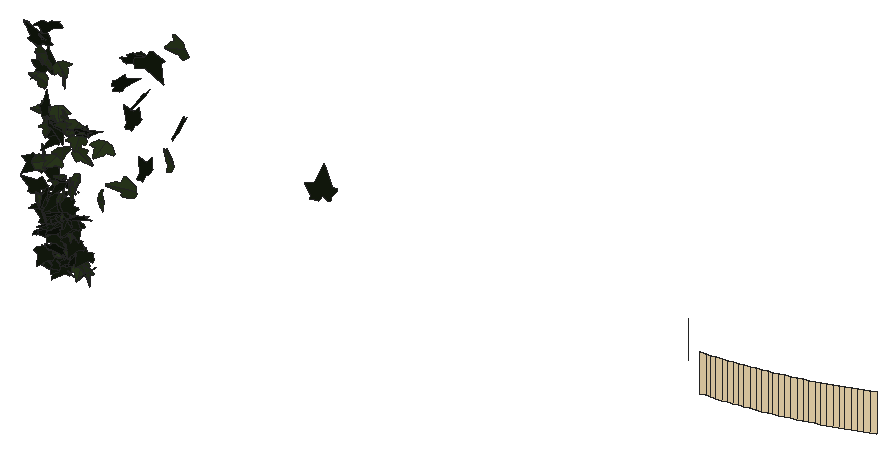
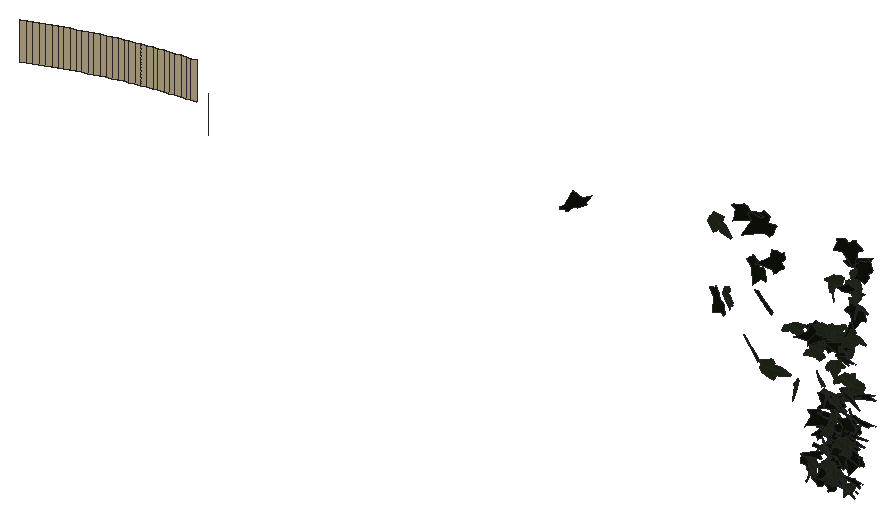
# SketchUp Ruby script. Lengths in inches.
U = 1.inch
M = Sketchup.active_model
def pt(a) = Geom::Point3d.new(a.map { |v| v * U })
def face(e, loops, mat)
  f = e.add_face(loops[0].map { |a| pt(a) })
  loops[1..].each { |l| e.add_face(l.map { |a| pt(a) }).erase! }
  f.material = f.back_material = mat if mat
  f
end
# faces: each face lists its corners as indices into pts; further lists are holes
def faces(e, pts, list, mat = nil) = list.each { |f| face(e, (f[0].is_a?(Array) ? f : [f]).map { |l| l.map { |i| pts[i] } }, mat) }
# xy, xz, yz: faces in a plane at the given z, y or x. An outline is a flat list of corners, or four numbers for a rectangle; further outlines are holes
def ring(l) = l.size == 4 ? [[l[0], l[1]], [l[2], l[1]], [l[2], l[3]], [l[0], l[3]]] : l.each_slice(2).to_a
def flat(e, list, mat, &to3) = list.each { |f| face(e, (f[0].is_a?(Array) ? f : [f]).map { |l| ring(l).map { |u, v| to3.(u, v) } }, mat) }
def xy(e, z, list, mat = nil) = flat(e, list, mat) { |x, y| [x, y, z] }
def xz(e, y, list, mat = nil) = flat(e, list, mat) { |x, z| [x, y, z] }
def yz(e, x, list, mat = nil) = flat(e, list, mat) { |y, z| [x, y, z] }
def lines(e, pts, list) = list.each { |a, b| e.add_line(pt(pts[a]), pt(pts[b])) }
# prism: a flat outline (further loops are holes) pulled along v
def prism(e, loops, v, mat = nil)
  f = face(e, loops, mat); d = Geom::Vector3d.new(v.map { |x| x * U })
  f.pushpull(f.normal.samedirection?(d) ? d.length : -d.length)
end
def box(e, o, s, mat = nil) = prism(e, [[o, [o[0] + s[0], o[1], o[2]], [o[0] + s[0], o[1] + s[1], o[2]], [o[0], o[1] + s[1], o[2]]]], [0, 0, s[2]], mat)
def at(x, y, z, deg = 0) = Geom::Transformation.translation(pt([x, y, z])) * Geom::Transformation.rotation(ORIGIN, Z_AXIS, deg.degrees)
def axes(o, x, y, z) = Geom::Transformation.new([*x, 0, *y, 0, *z, 0, *pt(o).to_a, 1])
def part(name) = M.definitions.add(name)
# library, detail: a bought-in or finely detailed component or shape, given as its bounding box
def library(name, o, s) = part(name).tap { |d| box(d.entities, o, s) }
def detail(e, o, s) = box(e.add_group.entities, o, s)
def put(e, d, t, mat = nil) = e.add_instance(d, t).tap { |i| i.material = mat if mat }
def group(e, t, mat = nil) = e.add_group.tap { |g| g.transformation = t; g.material = mat if mat }.entities
root = M.entities
M.materials.add("1026 AP 7946 SUNNY SIDE UP").color = [254, 231, 186]
M.materials.add("efeu1").color = [18, 25, 13]
M.materials.add("efeu2").color = [43, 57, 29]
c1 = part("ivyleaf_9")
p = [[1.54,2.16,1.25],[1.36,2.04,1.19],[-0.21,0.99,0.68],[-0.71,1.11,0.82],[-0.85,0.86,0.67],[-0.8,0.17,0.21],
  [-0.9,-0.01,0.1],[-0.67,-0.16,-0.02],[-0.08,-0.08,-0.05],[-0.03,-0.6,-0.4],[0.65,-0.88,-0.66],[0.83,-0.6,-0.49],
  [1.29,-0.42,-0.43],[1.8125,-0.07,-0.26],[1.21,0.44,0.15]]
faces(c1.entities,p,[[0,1,2,3,4,5,6,7,8,9,10,11,12,13,14]],"efeu1")
c2 = part("ivyleaf_10")
p = [[0,0.5,-0.03],[-0.0625,2.02,-0.43],[-0.19,2.01,-0.46],[-0.54,1.05,-0.29],[-0.52,0.625,-0.18],[-0.83,0.76,-0.28],
  [-1.16,0.64,-0.33],[-1.15,0.33,-0.24],[-0.77,-0.39,0.02],[-0.3,-0.51,0.16],[0.04,-0.48,0.23],[-0.02,2.01,-0.4375],
  [-0.06,2.01,-0.43],[0.04,-0.49,0.23],[0.67,-0.49,0.14],[1.38,0.36,-0.2],[1.375,0.51,-0.24],[0.81,0.65,-0.19],
  [0.62,0.59,-0.15],[0.6,1.09,-0.28],[0.5,1.23,-0.31]]
faces(c2.entities,p,[[0,1,2,3,4,5,6,7,8,9,10],[11,12,0,13,14,15,16,17,18,19,20]],"efeu2")
p = [[179.45,213.12,276],[179.18,213.09,276],[179.18,213.09,274],[179.45,213.12,274],[179.72,213.14,276],[179.72,213.14,274],
  [179.99,213.17,276],[179.99,213.17,274],[180.26,213.21,276],[180.26,213.21,274],[180.53,213.24,276],[180.53,213.24,274],
  [180.8,213.28,276],[180.8,213.28,274],[181.07,213.32,276],[181.07,213.32,274],[181.34,213.36,276],[181.34,213.36,274],
  [181.6,213.41,276],[181.6,213.41,274],[181.87,213.46,276],[181.87,213.46,274],[182.14,213.51,276],[182.14,213.51,274],
  [182.41,213.57,276],[182.41,213.57,274],[182.67,213.625,276],[182.67,213.625,274],[182.9375,213.6875,276],[182.9375,213.6875,274],
  [183.2,213.75,276],[183.2,213.75,274],[183.47,213.82,276],[183.47,213.82,274],[183.73,213.89,276],[183.73,213.89,274],
  [183.99,213.96,276],[183.99,213.96,274],[184.25,214.03,276],[184.25,214.03,274],[184.51,214.11,276],[184.51,214.11,274],
  [184.78,214.19,276],[184.78,214.19,274],[185.03,214.27,276],[185.03,214.27,274],[185.29,214.36,276],[185.29,214.36,274],
  [185.55,214.45,276],[185.55,214.45,274],[185.81,214.54,276],[185.81,214.54,274],[186.0625,214.63,276],[186.0625,214.63,274],
  [186.32,214.73,276],[186.32,214.73,274],[186.57,214.83,276],[186.57,214.83,274],[186.82,214.93,276],[186.82,214.93,274],
  [187.08,215.03,276],[187.08,215.03,274],[177,215,276],[177,215,274]]
faces(root,p,[[0,1,2,3],[4,0,3,5],[6,4,5,7],[8,6,7,9],[10,8,9,11],[12,10,11,13],[14,12,13,15],[16,14,15,17],
  [18,16,17,19],[20,18,19,21],[22,20,21,23],[24,22,23,25],[26,24,25,27],[28,26,27,29],[30,28,29,31],[32,30,31,33],
  [34,32,33,35],[36,34,35,37],[38,36,37,39],[40,38,39,41],[42,40,41,43],[44,42,43,45],[46,44,45,47],[48,46,47,49],
  [50,48,49,51],[52,50,51,53],[54,52,53,55],[56,54,55,57],[58,56,57,59],[60,58,59,61]],"1026 AP 7946 SUNNY SIDE UP")
lines(root,p,[[62,63]])
put(root,c1,axes([143.61,213.29,271.27],[-0.09913,0.13059,0.22675],[-0.33184,0.10048,-0.12352],[-0.22588,-0.20493,0.08196]),"1026 AP 7946 SUNNY SIDE UP")
put(root,c1,axes([143.49,213.3,272.49],[-0.32387,-0.14946,0.08965],[-0.08619,-0.07332,-0.26126],[0.25864,-0.21159,0.0252]),"1026 AP 7946 SUNNY SIDE UP")
put(root,c1,axes([142.99,213.43,278.64],[0.3595,-0.07239,-0.25962],[0.40076,-0.01486,0.24291],[-0.09416,-0.33964,0.04263]),"1026 AP 7946 SUNNY SIDE UP")
put(root,c1,axes([143.46,213.46,276.65],[0.09789,0.26986,0.09601],[0.03101,0.08952,-0.28478],[-0.44706,0.0653,0.00127]),"1026 AP 7946 SUNNY SIDE UP")
put(root,c2,axes([143.45,213.37,277.58],[-0.29524,0.23046,-0.01408],[-0.02661,-0.03298,-0.30443],[-0.36216,-0.18545,0.03385]),"1026 AP 7946 SUNNY SIDE UP")
put(root,c2,axes([143.61,213.39,276.51],[-0.21402,0.21849,0.14808],[-0.13843,0.11282,-0.26418],[-0.3861,-0.16156,0.01264]),"1026 AP 7946 SUNNY SIDE UP")
put(root,c2,axes([143.57,213.22,270.94],[-0.05715,0.25572,-0.04738],[0.00083,-0.04783,-0.26629],[-0.40895,-0.03583,0.00608]),"1026 AP 7946 SUNNY SIDE UP")
put(root,c1,axes([143.87,213.11,278.48],[0.14842,-0.05134,0.30276],[-0.36988,0.17727,0.11066],[-0.28925,-0.25303,0.01384]),"1026 AP 7946 SUNNY SIDE UP")
put(root,c2,axes([143.98,213.11,276.65],[0.01161,0.05816,0.30872],[-0.478,0.02489,0.00289],[-0.03761,-0.29839,0.05859]),"1026 AP 7946 SUNNY SIDE UP")
put(root,c2,axes([144.12,213.18,275.16],[-0.07558,0.03672,0.29561],[-0.45035,-0.04546,-0.04373],[0.06163,-0.28716,0.04298]),"1026 AP 7946 SUNNY SIDE UP")
put(root,c2,axes([143.87,213.23,273.22],[-0.24962,0.20753,0.10952],[-0.14861,0.05877,-0.26619],[-0.33426,-0.18111,0.03656]),"1026 AP 7946 SUNNY SIDE UP")
put(root,c2,axes([143.56,213.32,272.66],[0.18418,0.10926,0.2243],[0.25479,0.14452,-0.16414],[-0.28484,0.19992,-0.00179]),"1026 AP 7946 SUNNY SIDE UP")
put(root,c2,axes([144,213.22,277.64],[-0.35692,0.13818,0.15601],[-0.24653,0.0268,-0.26852],[-0.20628,-0.27111,0.05096]),"1026 AP 7946 SUNNY SIDE UP")
put(root,c2,axes([143.99,213.05,278.04],[0.2434,-0.08979,-0.24668],[-0.23685,0.19347,-0.1743],[0.32403,0.20887,0.0579]),"1026 AP 7946 SUNNY SIDE UP")
put(root,c1,axes([144.0625,213.53,270.61],[-0.36812,-0.03255,0.11188],[-0.15696,-0.05981,-0.2401],[0.0851,-0.25113,0.0411]),"1026 AP 7946 SUNNY SIDE UP")
put(root,c1,axes([143.76,213.375,271.04],[0.30535,0.16507,0.05638],[0.0115,0.07286,-0.25711],[-0.27275,0.18787,0.05228]),"1026 AP 7946 SUNNY SIDE UP")
put(root,c1,axes([143.82,213.19,269.35],[0.22382,0.21561,-0.00542],[0.01119,-0.01246,-0.26591],[-0.339,0.14194,-0.01235]),"1026 AP 7946 SUNNY SIDE UP")
put(root,c1,axes([144.07,213.52,272.6],[-0.26018,0.21373,-0.01225],[-0.00619,-0.0196,-0.27814],[-0.33665,-0.16482,0.01458]),"1026 AP 7946 SUNNY SIDE UP")
put(root,c2,axes([143.71,212.99,272.65],[-0.00374,-0.0192,0.2891],[0.12633,0.26901,0.02123],[-0.42404,0.08031,0.00377]),"1026 AP 7946 SUNNY SIDE UP")
put(root,c1,axes([144.23,213.14,270.14],[-0.12213,0.12558,0.23743],[-0.26875,0.15723,-0.14714],[-0.31189,-0.18466,0.03382]),"1026 AP 7946 SUNNY SIDE UP")
put(root,c1,axes([144.01,213.31,268.36],[-0.35977,-0.06867,-0.05982],[0.10001,-0.01283,-0.24426],[0.09941,-0.23561,0.02924]),"1026 AP 7946 SUNNY SIDE UP")
put(root,c2,axes([143.9,213.32,268.02],[0.09122,0.17682,0.1657],[-0.00235,0.16477,-0.18626],[-0.37479,0.042,0.0415]),"1026 AP 7946 SUNNY SIDE UP")
put(root,c1,axes([144,213.08,270.2],[0.21788,-0.06143,-0.22619],[-0.31602,0.08753,-0.15563],[0.16814,0.24412,0.00059]),"1026 AP 7946 SUNNY SIDE UP")
put(root,c2,axes([144.0625,213.36,275.07],[0.03687,0.26478,-0.1092],[-0.15451,-0.09382,-0.26068],[-0.42195,0.05749,0.08591]),"1026 AP 7946 SUNNY SIDE UP")
put(root,c1,axes([144.17,213.23,269.72],[-0.014,0.20216,-0.16617],[-0.0559,-0.16196,-0.20658],[-0.40394,0.01541,0.03435]),"1026 AP 7946 SUNNY SIDE UP")
put(root,c1,axes([144.12,213.19,277.23],[-0.44739,0.03099,0.09881],[0.15426,0.02153,0.29331],[0.03521,0.29943,-0.02954]),"1026 AP 7946 SUNNY SIDE UP")
put(root,c1,axes([143.99,213.22,271.34],[-0.2159,0.04529,-0.23582],[0.3143,-0.1148,-0.14742],[-0.1901,-0.24123,0.0241]),"1026 AP 7946 SUNNY SIDE UP")
put(root,c1,axes([144.18,213.15,279.48],[0.1907,0.23854,-0.14869],[-0.08354,-0.13624,-0.27617],[-0.43149,0.1318,-0.01225]),"1026 AP 7946 SUNNY SIDE UP")
put(root,c1,axes([144.05,213.53,270.56],[-0.19851,-0.22617,0.02611],[0.0683,-0.0538,-0.25893],[0.35151,-0.11727,0.06506]),"1026 AP 7946 SUNNY SIDE UP")
put(root,c2,axes([144.18,213.51,270.14],[-0.30747,-0.16306,0.03423],[-0.00848,-0.04645,-0.2605],[0.26182,-0.19299,0.03177]),"1026 AP 7946 SUNNY SIDE UP")
put(root,c1,axes([144.3,213.53,268.16],[-0.2948,0.1455,-0.04794],[0.03518,-0.04803,-0.24354],[-0.23802,-0.18731,0.02338]),"1026 AP 7946 SUNNY SIDE UP")
put(root,c1,axes([144.21,213.04,275.23],[-0.13172,-0.14288,0.25811],[0.16369,0.22923,0.17132],[-0.42413,0.13284,-0.01404]),"1026 AP 7946 SUNNY SIDE UP")
put(root,c2,axes([144.17,213.52,269.58],[0.19683,0.17099,-0.14619],[-0.10835,-0.12614,-0.21845],[-0.33319,0.14203,-0.01532]),"1026 AP 7946 SUNNY SIDE UP")
put(root,c1,axes([144.49,213.26,270.09],[-0.16447,0.19941,0.13415],[-0.19177,0.07595,-0.22224],[-0.32053,-0.14777,0.06413]),"1026 AP 7946 SUNNY SIDE UP")
put(root,c1,axes([144.33,213.56,269.68],[-0.00728,0.25296,-0.00825],[0.00227,-0.00942,-0.26069],[-0.39802,-0.00468,-0.00133]),"1026 AP 7946 SUNNY SIDE UP")
put(root,c2,axes([144.33,213.16,274.62],[-0.19373,-0.25873,0.07062],[-0.03153,-0.06795,-0.29541],[0.42028,-0.12436,0.01039]),"1026 AP 7946 SUNNY SIDE UP")
put(root,c1,axes([144.41,213.29,272.21],[-0.14668,-0.21709,0.15277],[0.07429,0.14227,0.244],[-0.40778,0.10401,-0.0105]),"1026 AP 7946 SUNNY SIDE UP")
put(root,c2,axes([144.47,213.23,273.02],[0.25979,0.13936,-0.17727],[-0.22972,-0.09404,-0.2225],[-0.26293,0.21986,0.01924]),"1026 AP 7946 SUNNY SIDE UP")
put(root,c1,axes([144.72,213.12,267.98],[-0.2552,0.15033,0.12111],[-0.17677,0.04803,-0.22452],[-0.24146,-0.19405,0.03636]),"1026 AP 7946 SUNNY SIDE UP")
put(root,c1,axes([144.27,213.22,274.38],[0.00556,0.01583,0.298],[0.41275,0.122,-0.00947],[-0.19238,0.26221,-0.01171]),"1026 AP 7946 SUNNY SIDE UP")
put(root,c1,axes([144.71,213.39,270.11],[-0.19778,0.2148,-0.07329],[-0.04597,-0.09744,-0.24619],[-0.35342,-0.10753,0.07304]),"1026 AP 7946 SUNNY SIDE UP")
put(root,c2,axes([144.51,213.59,268.6],[-0.08656,-0.22619,-0.0857],[0.03571,0.07876,-0.23933],[0.37656,-0.05946,0.003]),"1026 AP 7946 SUNNY SIDE UP")
put(root,c1,axes([144.63,213.29,274.08],[-0.39604,0.04034,-0.12276],[0.13362,-0.14267,-0.23518],[-0.14632,-0.23946,0.1175]),"1026 AP 7946 SUNNY SIDE UP")
put(root,c2,axes([144.79,213.37,274.84],[-0.28615,-0.0036,-0.22425],[-0.34103,-0.02137,0.18705],[-0.02941,0.28291,0.01294]),"1026 AP 7946 SUNNY SIDE UP")
put(root,c1,axes([144.73,213.44,271.83],[-0.33314,0.16492,-0.02738],[0.00923,-0.03705,-0.27556],[-0.26275,-0.21041,0.02504]),"1026 AP 7946 SUNNY SIDE UP")
put(root,c2,axes([144.56,213.38,272.07],[-0.19087,-0.24586,0.00486],[0.02712,-0.01531,-0.28163],[0.38576,-0.12057,0.0222]),"1026 AP 7946 SUNNY SIDE UP")
put(root,c1,axes([144.71,213.38,271],[-0.36721,-0.1088,0.07197],[-0.0797,-0.05701,-0.26403],[0.1876,-0.23718,0.02869]),"1026 AP 7946 SUNNY SIDE UP")
put(root,c1,axes([144.44,213.12,270.41],[0.25422,0.1867,0.09226],[0.12166,0.04948,-0.25288],[-0.30123,0.17755,-0.02427]),"1026 AP 7946 SUNNY SIDE UP")
put(root,c1,axes([144.8125,213.4,269.78],[-0.06089,-0.08955,-0.24798],[-0.18285,-0.21036,0.09888],[-0.35923,0.12225,-0.0083]),"1026 AP 7946 SUNNY SIDE UP")
put(root,c1,axes([144.47,213.46,269.18],[-0.14338,-0.18914,-0.13725],[0.15105,0.09808,-0.21232],[0.32987,-0.12712,0.03757]),"1026 AP 7946 SUNNY SIDE UP")
put(root,c1,axes([144.46,213.3,274.63],[0.05514,-0.27563,0.07187],[0.06665,-0.06601,-0.28464],[0.44269,0.04427,0.0339]),"1026 AP 7946 SUNNY SIDE UP")
put(root,c1,axes([144.64,212.96,269.76],[0.19418,0.21954,0.06131],[0.06406,0.04384,-0.25886],[-0.35137,0.12932,-0.01331]),"1026 AP 7946 SUNNY SIDE UP")
put(root,c2,axes([144.66,213.375,271.05],[-0.00465,0.14196,0.233],[-0.05323,0.22335,-0.14409],[-0.41542,-0.03021,0.01586]),"1026 AP 7946 SUNNY SIDE UP")
put(root,c2,axes([144.61,213.3,275.4],[0.23879,0.24488,-0.01844],[0.00344,-0.02403,-0.29662],[-0.38623,0.15119,-0.01404]),"1026 AP 7946 SUNNY SIDE UP")
put(root,c1,axes([144.95,213.05,268.15],[-0.06826,0.18588,0.16202],[-0.20933,0.11449,-0.17779],[-0.31928,-0.1148,0.08192]),"1026 AP 7946 SUNNY SIDE UP")
put(root,c1,axes([144.52,213.01,268.95],[0.39921,0.04935,0.01136],[0.02399,-0.02242,-0.26534],[-0.0757,0.25313,-0.02417]),"1026 AP 7946 SUNNY SIDE UP")
put(root,c1,axes([144.8,213.33,271.97],[-0.35928,0.07661,-0.1252],[0.16414,-0.06951,-0.24685],[-0.15605,-0.24951,0.02861]),"1026 AP 7946 SUNNY SIDE UP")
put(root,c1,axes([144.84,213.38,274.7],[-0.0122,0.09079,-0.27847],[-0.00875,-0.27092,-0.09498],[-0.44905,0.00281,0.00942]),"1026 AP 7946 SUNNY SIDE UP")
put(root,c1,axes([144.9,213.44,268.41],[-0.2658,0.17374,-0.05315],[0.01226,-0.06483,-0.2469],[-0.28516,-0.16473,0.03893]),"1026 AP 7946 SUNNY SIDE UP")
put(root,c2,axes([144.69,213.57,268.22],[0.34891,0.10471,-0.02297],[-0.03333,-0.00871,-0.25281],[-0.1652,0.2229,0.0025]),"1026 AP 7946 SUNNY SIDE UP")
put(root,c1,axes([144.99,213.44,268.37],[-0.26082,0.1893,0.03145],[-0.06033,0.00535,-0.25796],[-0.29514,-0.16838,0.02493]),"1026 AP 7946 SUNNY SIDE UP")
put(root,c1,axes([144.91,213.35,270.55],[-0.35437,0.11025,-0.07623],[0.09171,-0.05013,-0.25805],[-0.18817,-0.23205,0.0178]),"1026 AP 7946 SUNNY SIDE UP")
put(root,c1,axes([144.5,213.37,271.88],[0.39932,0.01387,0.09008],[0.13628,0.0141,-0.26177],[-0.02781,0.26819,0.01068]),"1026 AP 7946 SUNNY SIDE UP")
put(root,c2,axes([144.84,213.32,273.56],[-0.21172,-0.24372,-0.00624],[0.02548,-0.00362,-0.2864],[0.38245,-0.13468,0.01562]),"1026 AP 7946 SUNNY SIDE UP")
put(root,c1,axes([144.88,213.35,267.96],[-0.33884,-0.13001,0.00623],[0.00819,-0.02171,-0.25847],[0.20454,-0.2145,0.02066]),"1026 AP 7946 SUNNY SIDE UP")
put(root,c1,axes([144.57,213.54,267.89],[0.14368,-0.1773,0.14097],[0.15843,-0.10064,-0.20274],[0.31559,0.13124,0.0376]),"1026 AP 7946 SUNNY SIDE UP")
put(root,c2,axes([144.86,213.27,271.41],[0.06921,-0.18361,-0.20422],[0.02007,0.201,-0.1887],[0.42319,0.02049,0.04235]),"1026 AP 7946 SUNNY SIDE UP")
put(root,c2,axes([144.79,213.17,277.62],[0.18589,0.25742,0.12979],[-0.00296,0.13544,-0.28582],[-0.44963,0.10554,0.05554]),"1026 AP 7946 SUNNY SIDE UP")
put(root,c2,axes([144.83,213.41,275.26],[-0.26975,0.2132,-0.09298],[0.06655,-0.08309,-0.28178],[-0.35866,-0.17576,0.01764]),"1026 AP 7946 SUNNY SIDE UP")
put(root,c2,axes([144.88,213.43,268.82],[-0.28627,0.16887,-0.06227],[0.0558,-0.0519,-0.25574],[-0.27698,-0.18499,0.01284]),"1026 AP 7946 SUNNY SIDE UP")
put(root,c2,axes([144.77,213.45,277.02],[0.05935,-0.09106,0.28425],[0.3115,-0.19617,-0.09558],[0.33526,0.19839,0.03849]),"1026 AP 7946 SUNNY SIDE UP")
put(root,c1,axes([145.25,213.16,268.47],[-0.17863,0.21637,0.04323],[-0.09506,0.01341,-0.24705],[-0.33289,-0.11994,0.04736]),"1026 AP 7946 SUNNY SIDE UP")
put(root,c2,axes([144.97,213.43,270.43],[0.12406,0.24738,-0.02573],[-0.01139,-0.02538,-0.26764],[-0.39102,0.07923,-0.00037]),"1026 AP 7946 SUNNY SIDE UP")
put(root,c2,axes([145.07,213.53,268.69],[-0.3114,0.15448,0.00116],[-0.03839,-0.03091,-0.25573],[-0.23986,-0.19562,0.03943]),"1026 AP 7946 SUNNY SIDE UP")
put(root,c1,axes([145.31,213.34,271.02],[-0.39748,-0.0228,0.09403],[-0.13133,-0.06686,-0.25552],[0.06853,-0.26036,0.05575]),"1026 AP 7946 SUNNY SIDE UP")
put(root,c1,axes([144.88,213.29,270.78],[0.1417,-0.2496,0.04432],[0.01775,-0.04316,-0.27361],[0.39825,0.09074,-0.00358]),"1026 AP 7946 SUNNY SIDE UP")
put(root,c2,axes([144.85,213.4,268.88],[0.19412,-0.05665,0.22687],[0.31208,-0.09618,-0.14048],[0.17548,0.23373,-0.00114]),"1026 AP 7946 SUNNY SIDE UP")
put(root,c1,axes([145.36,213.3,270.13],[-0.38151,0.07708,0.04547],[-0.08739,-0.03316,-0.25781],[-0.10852,-0.24429,0.04775]),"1026 AP 7946 SUNNY SIDE UP")
put(root,c1,axes([145.17,213.54,268.19],[-0.20017,-0.08164,0.20057],[0.23004,0.13054,0.15534],[-0.24026,0.19301,-0.01838]),"1026 AP 7946 SUNNY SIDE UP")
put(root,c2,axes([145.04,213.53,269.48],[0.19031,-0.21641,-0.06273],[0.06582,-0.04484,0.25476],[-0.34679,-0.12727,0.01393]),"1026 AP 7946 SUNNY SIDE UP")
put(root,c1,axes([145.38,213.27,271.83],[-0.17609,0.24917,-0.03984],[0.00749,-0.04176,-0.28137],[-0.39676,-0.11137,0.01237]),"1026 AP 7946 SUNNY SIDE UP")
put(root,c2,axes([145.21,213.33,271.99],[0.10295,-0.1961,-0.192],[0.02929,0.19347,-0.20305],[0.42318,0.03431,0.06076]),"1026 AP 7946 SUNNY SIDE UP")
put(root,c2,axes([145.24,213.17,274.9],[-0.4276,-0.1065,-0.01751],[0.03807,-0.01705,-0.29989],[0.1651,-0.2719,0.02382]),"1026 AP 7946 SUNNY SIDE UP")
put(root,c2,axes([145.18,213.49,269.68],[0.05846,0.23997,-0.0777],[-0.01227,-0.07648,-0.25058],[-0.39598,0.0378,-0.00371]),"1026 AP 7946 SUNNY SIDE UP")
put(root,c1,axes([145.15,213.57,267.94],[0.25135,0.14779,0.11653],[-0.16479,-0.05041,0.22179],[0.24085,-0.18872,0.03015]),"1026 AP 7946 SUNNY SIDE UP")
put(root,c2,axes([145.26,213.3,271.97],[-0.31412,0.19115,-0.0235],[-0.03918,-0.05978,-0.27835],[-0.30036,-0.19211,0.06089]),"1026 AP 7946 SUNNY SIDE UP")
put(root,c1,axes([145.33,213.26,270.3125],[-0.34849,-0.12911,-0.03811],[0.10009,-0.03963,-0.25567],[0.1856,-0.22105,0.06632]),"1026 AP 7946 SUNNY SIDE UP")
put(root,c1,axes([145.35,213.375,270.21],[-0.05252,-0.24686,-0.09981],[0.02823,0.09391,-0.25603],[0.41523,-0.03761,0.00478]),"1026 AP 7946 SUNNY SIDE UP")
put(root,c2,axes([145.68,213.25,275.01],[-0.3675,-0.05323,0.17335],[-0.19008,-0.15578,-0.22424],[0.20282,-0.24243,0.10396]),"1026 AP 7946 SUNNY SIDE UP")
put(root,c1,axes([145.52,213.31,269.37],[-0.35176,-0.10493,-0.08254],[0.12888,0.01169,-0.25338],[0.162,-0.23713,0.02237]),"1026 AP 7946 SUNNY SIDE UP")
put(root,c2,axes([145.73,213.27,274.37],[-0.26581,-0.22435,0.07033],[0.01695,-0.093,-0.28264],[0.36894,-0.15736,0.06365]),"1026 AP 7946 SUNNY SIDE UP")
put(root,c2,axes([145.61,213.45,268.01],[0.37563,-0.06903,0.03654],[0.04267,-0.03459,-0.25503],[0.11464,0.23908,-0.02481]),"1026 AP 7946 SUNNY SIDE UP")
put(root,c1,axes([145.625,213.14,274.84],[0.38836,0.15405,0.01742],[-0.01479,0.04505,-0.2963],[-0.24309,0.24337,0.04586]),"1026 AP 7946 SUNNY SIDE UP")
put(root,c1,axes([145.64,213.1,270.63],[0.31125,0.1314,0.12572],[0.11366,0.10669,-0.23999],[-0.25718,0.20618,0.04609]),"1026 AP 7946 SUNNY SIDE UP")
put(root,c2,axes([145.71,213.2,272.57],[0.2924,-0.174,0.11526],[0.11802,-0.08486,-0.26266],[0.30401,0.2003,-0.00889]),"1026 AP 7946 SUNNY SIDE UP")
put(root,c1,axes([145.99,213.44,268.95],[-0.2797,-0.18013,0.03647],[-0.027,-0.03418,-0.26072],[0.28771,-0.17833,0.01099]),"1026 AP 7946 SUNNY SIDE UP")
put(root,c1,axes([145.74,213.3,274.6],[0.16242,0.10003,0.25933],[0.34123,0.12966,-0.14439],[-0.25351,0.23862,-0.0282]),"1026 AP 7946 SUNNY SIDE UP")
put(root,c2,axes([145.73,213.23,273.75],[0.23254,0.02995,0.24963],[0.36727,0.06447,-0.1548],[-0.1109,0.27631,0.01079]),"1026 AP 7946 SUNNY SIDE UP")
put(root,c2,axes([146.02,213.45,267.97],[-0.11449,0.23302,-0.05521],[0.02361,-0.05284,-0.25181],[-0.3757,-0.07433,0.001]),"1026 AP 7946 SUNNY SIDE UP")
put(root,c2,axes([145.95,213.39,268.43],[0.27187,-0.10986,0.15245],[0.23706,-0.03385,-0.20669],[0.16807,0.22546,0.04491]),"1026 AP 7946 SUNNY SIDE UP")
put(root,c2,axes([146.1875,213.14,268.41],[-0.38446,0.06141,-0.00648],[0.00101,-0.02456,-0.25871],[-0.09711,-0.24336,0.02295]),"1026 AP 7946 SUNNY SIDE UP")
put(root,c1,axes([146.42,213.02,268.33],[-0.03497,0.26692,0.00485],[-0.01101,0.00262,-0.27583],[-0.4196,-0.02231,0.00683]),"1026 AP 7946 SUNNY SIDE UP")
put(root,c2,axes([146.875,213.27,271.84],[-0.13999,0.18197,0.279],[-0.21824,0.23175,-0.20687],[-0.46282,-0.16432,0.01316]),"1026 AP 7946 SUNNY SIDE UP")
put(root,c2,axes([147.1,213.24,274.57],[0.38566,0.13717,-0.15653],[-0.18401,-0.10206,-0.28865],[-0.26519,0.2703,-0.02734]),"1026 AP 7946 SUNNY SIDE UP")
put(root,c2,axes([148.06,213.82,272.51],[-0.02959,0.01872,0.38127],[-0.52212,-0.16512,-0.00976],[0.25829,-0.33163,0.02395]),"1026 AP 7946 SUNNY SIDE UP")
put(root,c1,axes([147.63,213.47,277.53],[0.14288,0.10463,0.30712],[0.36153,0.18996,-0.14005],[-0.33945,0.24636,-0.01989]),"1026 AP 7946 SUNNY SIDE UP")
put(root,c1,axes([148.16,213.94,275.7],[-0.06435,0.16442,0.33143],[-0.17872,0.30049,-0.17185],[-0.53788,-0.11951,0.01745]),"1026 AP 7946 SUNNY SIDE UP")
put(root,c1,axes([148.67,214.08,273.39],[-0.06659,0.20745,0.33181],[-0.11512,0.31249,-0.21623],[-0.58973,-0.08442,0.00474]),"1026 AP 7946 SUNNY SIDE UP")
put(root,c1,axes([148.66,213.58,277.01],[0.06295,0.27645,0.27444],[0.04753,0.26316,-0.28617],[-0.60008,0.04984,0.00612]),"1026 AP 7946 SUNNY SIDE UP")
put(root,c1,axes([148.36,213.4,279.16],[0.47227,0.13828,0.11552],[0.17456,0.02449,-0.33967],[-0.21786,0.31939,-0.02174]),"1026 AP 7946 SUNNY SIDE UP")
put(root,c2,axes([149.93,214.94,279.44],[-0.25826,0.06132,0.37064],[-0.56556,0.03747,-0.17568],[-0.09413,-0.3934,0.03866]),"1026 AP 7946 SUNNY SIDE UP")
put(root,c1,axes([149.23,213.5,279.45],[-0.20763,-0.13923,-0.32368],[0.39571,0.1888,-0.19453],[0.36632,-0.28287,0.02668]),"1026 AP 7946 SUNNY SIDE UP")
put(root,c1,axes([149.86,214.71,275.51],[0.04579,0.20652,0.36264],[0.08018,0.34712,-0.21282],[-0.6351,0.05872,-0.00072]),"1026 AP 7946 SUNNY SIDE UP")
put(root,c2,axes([150.57,213.38,274.9],[-0.03901,0.00217,-0.4028],[-0.29424,0.34395,0.01621],[0.53986,0.18762,-0.02027]),"1026 AP 7946 SUNNY SIDE UP")
put(root,c1,axes([158.76,213.33,276.28],[-0.37854,-0.17803,0.29628],[0.32871,0.20077,0.3084],[-0.41983,0.31771,-0.02568]),"1026 AP 7946 SUNNY SIDE UP")
